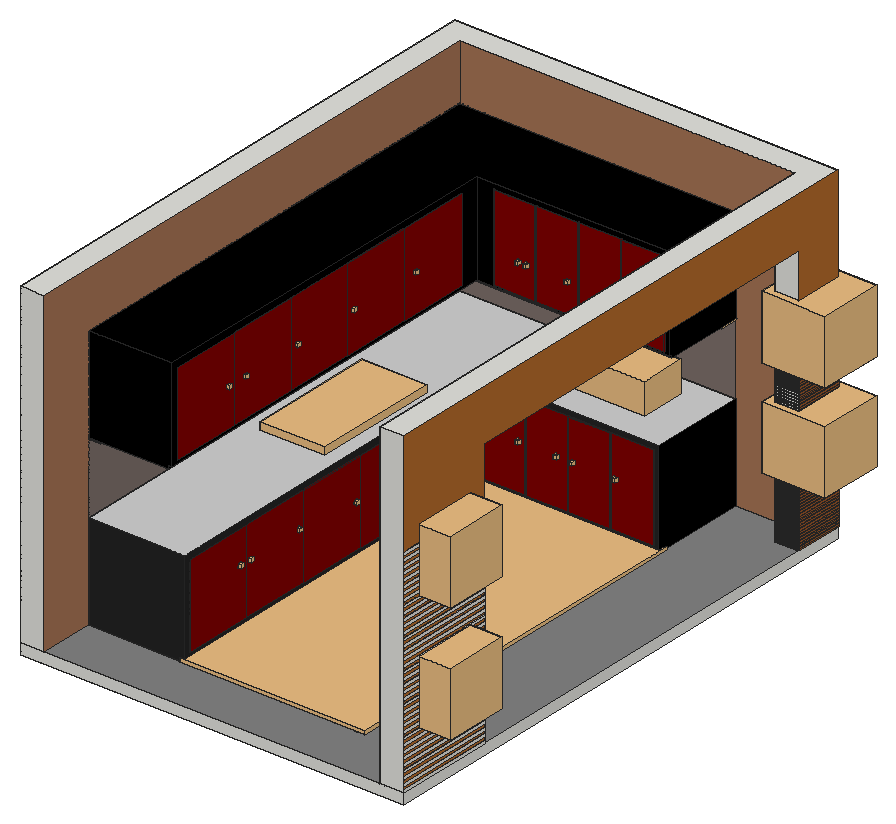
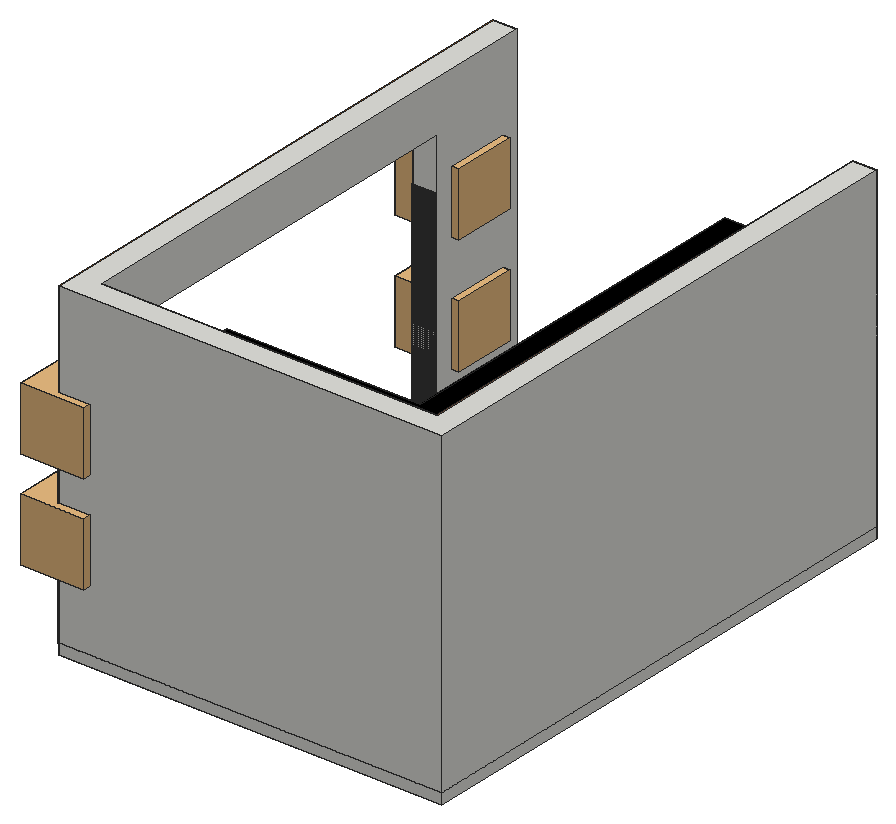
# SketchUp Ruby script. Lengths in inches.
U = 1.inch
M = Sketchup.active_model
def pt(a) = Geom::Point3d.new(a.map { |v| v * U })
def face(e, loops, mat)
  f = e.add_face(loops[0].map { |a| pt(a) })
  loops[1..].each { |l| e.add_face(l.map { |a| pt(a) }).erase! }
  f.material = f.back_material = mat if mat
  f
end
# faces: each face lists its corners as indices into pts; further lists are holes
def faces(e, pts, list, mat = nil) = list.each { |f| face(e, (f[0].is_a?(Array) ? f : [f]).map { |l| l.map { |i| pts[i] } }, mat) }
# xy, xz, yz: faces in a plane at the given z, y or x. An outline is a flat list of corners, or four numbers for a rectangle; further outlines are holes
def ring(l) = l.size == 4 ? [[l[0], l[1]], [l[2], l[1]], [l[2], l[3]], [l[0], l[3]]] : l.each_slice(2).to_a
def flat(e, list, mat, &to3) = list.each { |f| face(e, (f[0].is_a?(Array) ? f : [f]).map { |l| ring(l).map { |u, v| to3.(u, v) } }, mat) }
def xy(e, z, list, mat = nil) = flat(e, list, mat) { |x, y| [x, y, z] }
def xz(e, y, list, mat = nil) = flat(e, list, mat) { |x, z| [x, y, z] }
def yz(e, x, list, mat = nil) = flat(e, list, mat) { |y, z| [x, y, z] }
def lines(e, pts, list) = list.each { |a, b| e.add_line(pt(pts[a]), pt(pts[b])) }
# prism: a flat outline (further loops are holes) pulled along v
def prism(e, loops, v, mat = nil)
  f = face(e, loops, mat); d = Geom::Vector3d.new(v.map { |x| x * U })
  f.pushpull(f.normal.samedirection?(d) ? d.length : -d.length)
end
def box(e, o, s, mat = nil) = prism(e, [[o, [o[0] + s[0], o[1], o[2]], [o[0] + s[0], o[1] + s[1], o[2]], [o[0], o[1] + s[1], o[2]]]], [0, 0, s[2]], mat)
def at(x, y, z, deg = 0) = Geom::Transformation.translation(pt([x, y, z])) * Geom::Transformation.rotation(ORIGIN, Z_AXIS, deg.degrees)
def axes(o, x, y, z) = Geom::Transformation.new([*x, 0, *y, 0, *z, 0, *pt(o).to_a, 1])
def part(name) = M.definitions.add(name)
# library, detail: a bought-in or finely detailed component or shape, given as its bounding box
def library(name, o, s) = part(name).tap { |d| box(d.entities, o, s) }
def detail(e, o, s) = box(e.add_group.entities, o, s)
def put(e, d, t, mat = nil) = e.add_instance(d, t).tap { |i| i.material = mat if mat }
def group(e, t, mat = nil) = e.add_group.tap { |g| g.transformation = t; g.material = mat if mat }.entities
root = M.entities
M.materials.add("[0022_Maroon]").color = [128, 0, 0]
M.materials.add("[0136_Charcoal]").color = [35, 35, 35]
M.materials.add("[0137_Black]").color = [0, 0, 0]
M.materials.add("[Carrera Marble]").color = [207, 207, 207]
M.materials.add("[Herringbone]").color = [130, 130, 130]
M.materials.add("[Tile Ceramic Multi]").color = [165, 115, 84]
M.materials.add("[Tile Checker BW]").color = [125, 112, 107]
M.materials.add("[Wood Bamboo]").color = [177, 105, 43]
M.materials.add("[Wood Cherry Original]").color = [152, 86, 42]
c1 = part("Group\#10")
box(c1.entities,[0,0,0],[9,0.1875,0.36])
c2 = part("Group\#16")
box(c2.entities,[0,0,0],[0.125,18.33,0.46])
c3 = library("Group\#20",[-0.5,-0.5,0],[69.68,141.4375,1.125])
c4 = part("Group\#8")
box(c4.entities,[0,0,0],[0.25,37.84,0.98])
c5 = part("Group\#5")
xy(c5.entities,0,[[0,0,15.73,0.28],[16,0,31.73,0.28],[32.01,0,47.74,0.28],[48.01,0,64.02,0.28]])
xy(c5.entities,32.22,[[0,0,15.73,0.28],[16,0,31.73,0.28],[32.01,0,47.74,0.28],[48.01,0,64.02,0.28]])
xz(c5.entities,0,[[0,0,15.73,32.22],[16,0,31.73,32.22],[32.01,0,47.74,32.22],[48.01,0,64.02,32.22]])
xz(c5.entities,0.28,[[0,0,15.73,32.22],[15.73,0,16,32.22],[16,0,31.73,32.22],[31.73,0,32.01,32.22],[32.01,0,47.74,32.22],
  [47.74,0,48.01,32.22],[48.01,0,64.02,32.22]])
yz(c5.entities,0,[[0,0,0.28,32.22]])
yz(c5.entities,15.73,[[0,0,0.28,32.22]])
yz(c5.entities,16,[[0,0,0.28,32.22]])
yz(c5.entities,31.73,[[0,0,0.28,32.22]])
yz(c5.entities,32.01,[[0,0,0.28,32.22]])
yz(c5.entities,47.74,[[0,0,0.28,32.22]])
yz(c5.entities,48.01,[[0,0,0.28,32.22]])
yz(c5.entities,64.02,[[0,0,0.28,32.22]])
c6 = part("Group\#4")
xy(c6.entities,0,[[0,0,0.28,26.15],[0,26.625,0.28,52.78],[0,53.25,0.28,79.4],[0,79.87,0.28,106.02],[0,106.5,0.28,133.12]])
xy(c6.entities,30.9375,[[0,0,0.28,26.15],[0,26.625,0.28,52.78],[0,53.25,0.28,79.4],[0,79.87,0.28,106.02],[0,106.5,0.28,133.12]])
xz(c6.entities,0,[[0,0,0.28,30.9375]])
xz(c6.entities,26.15,[[0,0,0.28,30.9375]])
xz(c6.entities,26.625,[[0,0,0.28,30.9375]])
xz(c6.entities,52.78,[[0,0,0.28,30.9375]])
xz(c6.entities,53.25,[[0,0,0.28,30.9375]])
xz(c6.entities,79.4,[[0,0,0.28,30.9375]])
xz(c6.entities,79.87,[[0,0,0.28,30.9375]])
xz(c6.entities,106.02,[[0,0,0.28,30.9375]])
xz(c6.entities,106.5,[[0,0,0.28,30.9375]])
xz(c6.entities,133.12,[[0,0,0.28,30.9375]])
yz(c6.entities,0,[[0,0,26.15,30.9375],[26.15,0,26.625,30.9375],[26.625,0,52.78,30.9375],[52.78,0,53.25,30.9375],[53.25,0,79.4,30.9375],
  [79.4,0,79.87,30.9375],[79.87,0,106.02,30.9375],[106.02,0,106.5,30.9375],[106.5,0,133.12,30.9375]])
yz(c6.entities,0.28,[[0,0,26.15,30.9375],[26.625,0,52.78,30.9375],[53.25,0,79.4,30.9375],[79.87,0,106.02,30.9375],[106.5,0,133.12,30.9375]])
c7 = library("77459",[-0.64,-1.24,-0.66],[1.28,1.25,1.29])
c8 = library("Omni Light\#1",[-12,-12,-12],[24,24,24])
c9 = library("Omni Light\#3",[-12,-12,-12],[24,24,24])
c10 = library("Component_12",[0,0,0],[17.72,31.5,20.63])
c11 = library("Gas cooktop",[0,0,34.52],[24.41,48.07,2.63])
c12 = library("Omni Light\#2",[-12,-12,-12],[24,24,24])
c13 = library("Group\#18",[-0.5,-0.5,-0.1],[5.6,175.1875,0.2])
c14 = library("Group\#19",[-0.5,-0.5,-0.1],[99.7,7.49,0.2])
c15 = library("Omni Light",[-12,-12,-12],[24,24,24])
g1 = group(root,at(0,0,-4))
xy(g1,0,[[0,0,144,204]])
xy(g1,4,[[0,0,144,204]],"[Herringbone]")
xz(g1,0,[[0,0,144,4]])
xz(g1,204,[[0,0,144,4]])
yz(g1,0,[[0,0,204,4]])
yz(g1,144,[[0,0,204,4]])
put(root,c1,at(135,185.48,0))
put(root,c2,at(144,185.67,0),"[Wood Cherry Original]")
g2 = group(root,at(9,20.8125,0),"[0137_Black]")
xy(g2,0,[[0,0,0,174.1875,103.8,174.1875,103.8,140.4375,35.125,140.4375,35.125,0]])
xy(g2,1.125,[[35.125,0,36,140.4375],[36,138.1875,103.8,140.4375]])
xy(g2,1.89,[[37.89,138.1875,101.91,164.5625]])
xy(g2,2.53,[[9.625,2.53,36,135.65]])
xy(g2,33.47,[[9.625,2.53,36,135.65]])
xy(g2,34.11,[[37.89,138.1875,37.89,164.5625,57.61,164.5625,57.61,150.2,80.17,150.2,80.17,164.5625,101.91,164.5625,101.91,138.1875]])
xy(g2,34.11,[[57.61,164.5625,80.17,164.58]],"[Carrera Marble]")
xy(g2,36,[[[0,0,36,0,36,138.1875,103.8,138.1875,103.8,174.1875,0,174.1875],[57.61,150.2,80.17,164.58]]],"[Carrera Marble]")
xz(g2,0,[[0,0,35.125,0,35.125,1.125,36,1.125,36,36,0,36]],"[0136_Charcoal]")
xz(g2,2.53,[[9.625,2.53,36,33.47]])
xz(g2,135.65,[[9.625,2.53,36,33.47]])
xz(g2,138.1875,[[[36,1.125,103.8,36],[37.89,1.89,101.91,34.11]]],"[0136_Charcoal]")
xz(g2,150.2,[[57.61,34.11,80.17,36]],"[Carrera Marble]")
xz(g2,164.5625,[[37.89,1.89,101.91,34.11]])
xz(g2,164.58,[[57.61,34.11,80.17,36]],"[Carrera Marble]")
xz(g2,174.1875,[[0,0,103.8,36]])
yz(g2,0,[[0,0,174.1875,36]])
yz(g2,9.625,[[2.53,2.53,135.65,33.47]])
yz(g2,36,[[[0,1.125,138.1875,36],[2.53,2.53,135.65,33.47]]],"[0136_Charcoal]")
yz(g2,37.89,[[138.1875,1.89,164.5625,34.11]])
yz(g2,57.61,[[150.2,34.11,164.58,36]],"[Carrera Marble]")
yz(g2,80.17,[[150.2,34.11,164.58,36]],"[Carrera Marble]")
yz(g2,101.91,[[138.1875,1.89,164.5625,34.11]])
yz(g2,103.8,[[140.4375,0,174.1875,0,174.1875,36,138.1875,36,138.1875,1.125,140.4375,1.125]])
p = [[104.24,138.1875,1.125],[103.8,138.1875,1.125]]
lines(g2,p,[[0,1]])
put(g2,c3,at(35.125,0,0))
put(root,c4,at(144,0,0))
g3 = group(root,at(0,0,0))
xy(g3,0,[[0,0,0,204,144,204,144,185.67,135,185.67,135,195,9,195,9,0],[135,0,144,37.84]])
xy(g3,101.01,[[135,37.84,144,185.67]])
xy(g3,120,[[0,0,9,0,9,195,135,195,135,0,144,0,144,204,0,204]])
xz(g3,0,[[0,0,9,120],[135,0,144,120]])
xz(g3,37.84,[[135,0,144,101.01]])
xz(g3,185.67,[[135,0,144,101.01]])
xz(g3,195,[[9,0,135,0,135,120,9,120,9,63.0625,112.8,63.0625,112.8,36,9,36]],"[Tile Ceramic Multi]")
xz(g3,195,[[9,36,112.8,63.0625]],"[Tile Checker BW]")
xz(g3,204,[[0,0,144,120]])
yz(g3,0,[[0,0,204,120]])
yz(g3,9,[[0,0,195,0,195,36,20.8125,36,20.8125,63.0625,195,63.0625,195,120,0,120]],"[Tile Ceramic Multi]")
yz(g3,9,[[20.8125,36,195,63.0625]],"[Tile Checker BW]")
yz(g3,135,[[0,0,0,120,195,120,195,0,185.67,0,185.67,101.01,37.84,101.01,37.84,0]])
yz(g3,144,[[0,0,37.84,0,37.84,101.01,185.67,101.01,185.67,0,204,0,204,120,0,120]],"[Wood Bamboo]")
put(root,c1,at(135,37.84,0))
put(root,c2,at(144,185.67,0.5),"[Wood Cherry Original]")
put(root,c1,at(135,185.48,0.5))
put(root,c1,at(135,37.84,0.67))
put(root,c2,at(144,185.67,1.01),"[Wood Cherry Original]")
put(root,c1,at(135,185.48,1.01))
put(root,c1,at(135,37.84,1.34))
put(root,c2,at(144,185.67,1.51),"[Wood Cherry Original]")
put(root,c1,at(135,185.48,1.51))
put(root,c5,at(46.89,158.72,1.89),"[0022_Maroon]")
put(root,c2,at(144,185.67,2.01),"[Wood Cherry Original]")
put(root,c1,at(135,185.48,2.01))
put(root,c1,at(135,37.84,2.01))
put(root,c4,at(144,0,2.22))
put(root,c2,at(144,185.67,2.51),"[Wood Cherry Original]")
put(root,c1,at(135,185.48,2.52))
put(root,c6,at(45,23.35,2.53),"[0022_Maroon]")
put(root,c1,at(135,37.84,2.68))
put(root,c2,at(144,185.67,3.02),"[Wood Cherry Original]")
put(root,c1,at(135,185.48,3.02))
put(root,c1,at(135,37.84,3.35))
put(root,c2,at(144,185.67,3.52),"[Wood Cherry Original]")
put(root,c1,at(135,185.48,3.52))
put(root,c2,at(144,185.67,4.02),"[Wood Cherry Original]")
put(root,c1,at(135,185.48,4.03))
put(root,c1,at(135,37.84,4.03))
put(root,c4,at(144,0,4.44))
put(root,c2,at(144,185.67,4.52),"[Wood Cherry Original]")
put(root,c1,at(135,185.48,4.53))
put(root,c1,at(135,37.84,4.7))
put(root,c2,at(144,185.67,5.03),"[Wood Cherry Original]")
put(root,c1,at(135,185.48,5.03))
put(root,c1,at(135,37.84,5.37))
put(root,c2,at(144,185.67,5.53),"[Wood Cherry Original]")
put(root,c1,at(135,185.48,5.54))
put(root,c2,at(144,185.67,6.03),"[Wood Cherry Original]")
put(root,c1,at(135,185.48,6.04))
put(root,c1,at(135,37.84,6.04))
put(root,c2,at(144,185.67,6.54),"[Wood Cherry Original]")
put(root,c1,at(135,185.48,6.54))
put(root,c4,at(144,0,6.67))
put(root,c1,at(135,37.84,6.71))
put(root,c2,at(144,185.67,7.04),"[Wood Cherry Original]")
put(root,c1,at(135,185.48,7.05))
put(root,c1,at(135,37.84,7.38))
put(root,c2,at(144,185.67,7.54),"[Wood Cherry Original]")
put(root,c1,at(135,185.48,7.55))
put(root,c2,at(144,185.67,8.04),"[Wood Cherry Original]")
put(root,c1,at(135,185.48,8.05))
put(root,c1,at(135,37.84,8.05))
put(root,c2,at(144,185.67,8.55),"[Wood Cherry Original]")
put(root,c1,at(135,185.48,8.56))
put(root,c1,at(135,37.84,8.72))
put(root,c4,at(144,0,8.89))
put(root,c2,at(144,185.67,9.05),"[Wood Cherry Original]")
put(root,c1,at(135,185.48,9.06))
put(root,c1,at(135,37.84,9.39))
put(root,c2,at(144,185.67,9.55),"[Wood Cherry Original]")
put(root,c1,at(135,185.48,9.5625))
put(root,c2,at(144,185.67,10.05),"[Wood Cherry Original]")
put(root,c1,at(135,185.48,10.06))
put(root,c1,at(135,37.84,10.06))
put(root,c2,at(144,185.67,10.56),"[Wood Cherry Original]")
put(root,c1,at(135,185.48,10.57))
put(root,c1,at(135,37.84,10.74))
put(root,c2,at(144,185.67,11.06),"[Wood Cherry Original]")
put(root,c1,at(135,185.48,11.07))
put(root,c4,at(144,0,11.11))
put(root,c1,at(135,37.84,11.41))
put(root,c2,at(144,185.67,11.5625),"[Wood Cherry Original]")
put(root,c1,at(135,185.48,11.57))
put(root,c2,at(144,185.67,12.07),"[Wood Cherry Original]")
put(root,c1,at(135,185.48,12.08))
put(root,c1,at(135,37.84,12.08))
put(root,c2,at(144,185.67,12.57),"[Wood Cherry Original]")
put(root,c1,at(135,185.48,12.58))
put(root,c1,at(135,37.84,12.75))
put(root,c2,at(144,185.67,13.07),"[Wood Cherry Original]")
put(root,c1,at(135,185.48,13.08))
put(root,c4,at(144,0,13.33))
put(root,c1,at(135,37.84,13.42))
put(root,c2,at(144,185.67,13.57),"[Wood Cherry Original]")
put(root,c1,at(135,185.48,13.59))
put(root,c2,at(144,185.67,14.08),"[Wood Cherry Original]")
put(root,c1,at(135,185.48,14.09))
put(root,c1,at(135,37.84,14.09))
put(root,c2,at(144,185.67,14.58),"[Wood Cherry Original]")
put(root,c1,at(135,185.48,14.59))
put(root,c1,at(135,37.84,14.76))
put(root,c2,at(144,185.67,15.08),"[Wood Cherry Original]")
put(root,c1,at(135,185.48,15.1))
put(root,c1,at(135,37.84,15.43))
put(root,c4,at(144,0,15.56))
put(root,c2,at(144,185.67,15.59),"[Wood Cherry Original]")
put(root,c1,at(135,185.48,15.6))
put(root,c2,at(144,185.67,16.09),"[Wood Cherry Original]")
put(root,c1,at(135,185.48,16.1))
put(root,c1,at(135,37.84,16.1))
put(root,c2,at(144,185.67,16.59),"[Wood Cherry Original]")
put(root,c1,at(135,185.48,16.61))
put(root,c1,at(135,37.84,16.77))
put(root,c2,at(144,185.67,17.09),"[Wood Cherry Original]")
put(root,c1,at(135,185.48,17.11))
put(root,c1,at(135,37.84,17.45))
put(root,c2,at(144,185.67,17.6),"[Wood Cherry Original]")
put(root,c1,at(135,185.48,17.61))
put(root,c4,at(144,0,17.78))
put(root,c7,at(45.4375,128.42,18.74,90))
put(root,c7,at(45.4375,132.36,18.74,90))
put(root,c2,at(144,185.67,18.1),"[Wood Cherry Original]")
put(root,c1,at(135,185.48,18.12))
put(root,c1,at(135,37.84,18.12))
put(root,c7,at(45.29,100.7,19.2,90))
put(root,c2,at(144,185.67,18.6),"[Wood Cherry Original]")
put(root,c1,at(135,185.48,18.62))
put(root,c7,at(96.75,158.72,19.43))
put(root,c7,at(74.75,158.72,19.43))
put(root,c7,at(80.68,158.72,19.43))
put(root,c7,at(60.43,158.72,19.43))
put(root,c1,at(135,37.84,18.79))
put(root,c2,at(144,185.67,19.1),"[Wood Cherry Original]")
put(root,c8,at(144.25,18.92,31.11))
put(root,c1,at(135,185.48,19.125))
put(root,c1,at(135,37.84,19.46))
put(root,c2,at(144,185.67,19.61),"[Wood Cherry Original]")
put(root,c1,at(135,185.48,19.625))
put(root,c4,at(144,0,20))
put(root,c2,at(144,185.67,20.11),"[Wood Cherry Original]")
put(root,c1,at(135,185.48,20.13))
put(root,c1,at(135,37.84,20.13))
put(root,c2,at(144,185.67,20.61),"[Wood Cherry Original]")
put(root,c1,at(135,185.48,20.63))
put(root,c1,at(135,37.84,20.8))
put(root,c2,at(144,185.67,21.12),"[Wood Cherry Original]")
put(root,c1,at(135,185.48,21.14))
put(root,c7,at(45.29,73.71,21.81,90))
put(root,c7,at(45.29,50.96,21.81,90))
put(root,c7,at(45.29,46.33,21.81,90))
put(root,c1,at(135,37.84,21.47))
put(root,c2,at(144,185.67,21.62),"[Wood Cherry Original]")
put(root,c1,at(135,185.48,21.64))
put(root,c2,at(144,185.67,22.12),"[Wood Cherry Original]")
put(root,c1,at(135,185.48,22.14))
put(root,c1,at(135,37.84,22.14))
put(root,c4,at(144,0,22.22))
put(root,c2,at(144,185.67,22.625),"[Wood Cherry Original]")
put(root,c1,at(135,185.48,22.65))
put(root,c1,at(135,37.84,22.8125))
put(root,c2,at(144,185.67,23.125),"[Wood Cherry Original]")
put(root,c1,at(135,185.48,23.15))
put(root,c9,at(144.125,194.83,35.15))
put(root,c1,at(135,37.84,23.48))
put(root,c2,at(144,185.67,23.63),"[Wood Cherry Original]")
put(root,c1,at(135,185.48,23.65))
put(root,c2,at(144,185.67,24.13),"[Wood Cherry Original]")
put(root,c1,at(135,185.48,24.16))
put(root,c1,at(135,37.84,24.16))
put(root,c4,at(144,0,24.44))
put(root,c2,at(144,185.67,24.63),"[Wood Cherry Original]")
put(root,c1,at(135,185.48,24.66))
put(root,c1,at(135,37.84,24.83))
put(root,c2,at(144,185.67,25.14),"[Wood Cherry Original]")
put(root,c1,at(135,185.48,25.16))
put(root,c1,at(135,37.84,25.5))
put(root,c2,at(144,185.67,25.64),"[Wood Cherry Original]")
put(root,c1,at(135,185.48,25.67))
put(root,c2,at(144,185.67,26.14),"[Wood Cherry Original]")
put(root,c1,at(135,185.48,26.17))
put(root,c1,at(135,37.84,26.17))
put(root,c2,at(144,185.67,26.65),"[Wood Cherry Original]")
put(root,c4,at(144,0,26.67))
put(root,c1,at(135,185.48,26.67))
put(root,c1,at(135,37.84,26.84))
put(root,c10,axes([66.6,187.4375,26.92],[0,-0.96,0],[1,0,0],[0,0,1]))
put(root,c2,at(144,185.67,27.15),"[Wood Cherry Original]")
put(root,c1,at(135,185.48,27.18))
put(root,c1,at(135,37.84,27.51))
put(root,c2,at(144,185.67,27.65),"[Wood Cherry Original]")
put(root,c1,at(135,185.48,27.68))
put(root,c2,at(144,185.67,28.15),"[Wood Cherry Original]")
put(root,c1,at(135,185.48,28.18))
put(root,c1,at(135,37.84,28.18))
put(root,c2,at(144,185.67,28.66),"[Wood Cherry Original]")
put(root,c1,at(135,185.48,28.68))
put(root,c1,at(135,37.84,28.85))
put(root,c4,at(144,0,28.89))
put(root,c2,at(144,185.67,29.16),"[Wood Cherry Original]")
put(root,c1,at(135,185.48,29.1875))
put(root,c1,at(135,37.84,29.52))
put(root,c2,at(144,185.67,29.66),"[Wood Cherry Original]")
put(root,c1,at(135,185.48,29.69))
put(root,c2,at(144,185.67,30.16),"[Wood Cherry Original]")
put(root,c1,at(135,185.48,30.19))
put(root,c1,at(135,37.84,30.19))
put(root,c2,at(144,185.67,30.67),"[Wood Cherry Original]")
put(root,c1,at(135,185.48,30.7))
put(root,c1,at(135,37.84,30.87))
put(root,c4,at(144,0,31.11))
put(root,c2,at(144,185.67,31.17),"[Wood Cherry Original]")
put(root,c1,at(135,185.48,31.2))
put(root,c1,at(135,37.84,31.54))
put(root,c2,at(144,185.67,31.67),"[Wood Cherry Original]")
put(root,c1,at(135,185.48,31.7))
put(root,c2,at(144,185.67,32.18),"[Wood Cherry Original]")
put(root,c1,at(135,185.48,32.21))
put(root,c1,at(135,37.84,32.21))
put(root,c2,at(144,185.67,32.68),"[Wood Cherry Original]")
put(root,c1,at(135,185.48,32.71))
put(root,c1,at(135,37.84,32.88))
put(root,c2,at(144,185.67,33.18),"[Wood Cherry Original]")
put(root,c1,at(135,185.48,33.21))
put(root,c4,at(144,0,33.33))
put(root,c1,at(135,37.84,33.55))
put(root,c2,at(144,185.67,33.68),"[Wood Cherry Original]")
put(root,c1,at(135,185.48,33.72))
put(root,c2,at(144,185.67,34.1875),"[Wood Cherry Original]")
put(root,c1,at(135,37.84,34.22))
put(root,c1,at(135,185.48,34.22))
put(root,c2,at(144,185.67,34.6875),"[Wood Cherry Original]")
put(root,c1,at(135,185.48,34.72))
put(root,c1,at(135,37.84,34.89))
put(root,c2,at(144,185.67,35.19),"[Wood Cherry Original]")
put(root,c1,at(135,185.48,35.23))
put(root,c4,at(144,0,35.56))
put(root,c1,at(135,37.84,35.5625))
put(root,c2,at(144,185.67,35.69),"[Wood Cherry Original]")
put(root,c1,at(135,185.48,35.73))
put(root,c11,at(15.19,93.4,1.48))
put(root,c2,at(144,185.67,36.2),"[Wood Cherry Original]")
put(root,c1,at(135,37.84,36.23))
put(root,c1,at(135,185.48,36.23))
put(root,c2,at(144,185.67,36.7),"[Wood Cherry Original]")
put(root,c1,at(135,185.48,36.74))
put(root,c1,at(135,37.84,36.9))
put(root,c2,at(144,185.67,37.2),"[Wood Cherry Original]")
put(root,c1,at(135,185.48,37.24))
put(root,c1,at(135,37.84,37.58))
put(root,c2,at(144,185.67,37.71),"[Wood Cherry Original]")
put(root,c1,at(135,185.48,37.74))
put(root,c4,at(144,0,37.78))
put(root,c2,at(144,185.67,38.21),"[Wood Cherry Original]")
put(root,c1,at(135,37.84,38.25))
put(root,c1,at(135,185.48,38.25))
put(root,c2,at(144,185.67,38.71),"[Wood Cherry Original]")
put(root,c1,at(135,185.48,38.75))
put(root,c1,at(135,37.84,38.92))
put(root,c2,at(144,185.67,39.21),"[Wood Cherry Original]")
put(root,c1,at(135,185.48,39.25))
put(root,c1,at(135,37.84,39.59))
put(root,c2,at(144,185.67,39.72),"[Wood Cherry Original]")
put(root,c1,at(135,185.48,39.76))
put(root,c4,at(144,0,40))
put(root,c2,at(144,185.67,40.22),"[Wood Cherry Original]")
put(root,c1,at(135,37.84,40.26))
put(root,c1,at(135,185.48,40.26))
put(root,c2,at(144,185.67,40.72),"[Wood Cherry Original]")
put(root,c1,at(135,185.48,40.76))
put(root,c1,at(135,37.84,40.93))
put(root,c2,at(144,185.67,41.23),"[Wood Cherry Original]")
put(root,c1,at(135,185.48,41.27))
put(root,c1,at(135,37.84,41.6))
put(root,c2,at(144,185.67,41.73),"[Wood Cherry Original]")
put(root,c1,at(135,185.48,41.77))
put(root,c4,at(144,0,42.22))
put(root,c2,at(144,185.67,42.23),"[Wood Cherry Original]")
put(root,c1,at(135,37.84,42.27))
put(root,c1,at(135,185.48,42.27))
put(root,c2,at(144,185.67,42.73),"[Wood Cherry Original]")
put(root,c1,at(135,185.48,42.78))
put(root,c1,at(135,37.84,42.94))
put(root,c2,at(144,185.67,43.24),"[Wood Cherry Original]")
put(root,c1,at(135,185.48,43.28))
put(root,c1,at(135,37.84,43.61))
put(root,c2,at(144,185.67,43.74),"[Wood Cherry Original]")
put(root,c1,at(135,185.48,43.78))
put(root,c2,at(144,185.67,44.24),"[Wood Cherry Original]")
put(root,c1,at(135,37.84,44.29))
put(root,c1,at(135,185.48,44.29))
put(root,c4,at(144,0,44.44))
put(root,c2,at(144,185.67,44.74),"[Wood Cherry Original]")
put(root,c1,at(135,185.48,44.79))
put(root,c1,at(135,37.84,44.96))
put(root,c2,at(144,185.67,45.25),"[Wood Cherry Original]")
put(root,c1,at(135,185.48,45.29))
put(root,c1,at(135,37.84,45.63))
put(root,c2,at(144,185.67,45.75),"[Wood Cherry Original]")
put(root,c1,at(135,185.48,45.8))
put(root,c2,at(144,185.67,46.25),"[Wood Cherry Original]")
put(root,c1,at(135,37.84,46.3))
put(root,c1,at(135,185.48,46.3))
put(root,c4,at(144,0,46.67))
put(root,c2,at(144,185.67,46.76),"[Wood Cherry Original]")
put(root,c1,at(135,185.48,46.8))
put(root,c1,at(135,37.84,46.97))
put(root,c2,at(144,185.67,47.26),"[Wood Cherry Original]")
put(root,c1,at(135,185.48,47.3))
put(root,c1,at(135,37.84,47.64))
put(root,c2,at(144,185.67,47.76),"[Wood Cherry Original]")
put(root,c1,at(135,185.48,47.81))
put(root,c2,at(144,185.67,48.26),"[Wood Cherry Original]")
put(root,c1,at(135,37.84,48.3125))
put(root,c1,at(135,185.48,48.3125))
put(root,c2,at(144,185.67,48.77),"[Wood Cherry Original]")
put(root,c1,at(135,185.48,48.81))
put(root,c4,at(144,0,48.89))
put(root,c1,at(135,37.84,48.98))
put(root,c2,at(144,185.67,49.27),"[Wood Cherry Original]")
put(root,c1,at(135,185.48,49.32))
put(root,c1,at(135,37.84,49.65))
put(root,c2,at(144,185.67,49.77),"[Wood Cherry Original]")
put(root,c1,at(135,185.48,49.82))
put(root,c2,at(144,185.67,50.27),"[Wood Cherry Original]")
put(root,c1,at(135,37.84,50.32))
put(root,c1,at(135,185.48,50.32))
put(root,c2,at(144,185.67,50.78),"[Wood Cherry Original]")
put(root,c1,at(135,185.48,50.83))
put(root,c1,at(135,37.84,51))
put(root,c4,at(144,0,51.11))
g4 = group(root,at(144,185.67,51.28),"[Wood Cherry Original]")
box(g4,[0,0,0],[0.125,18.33,0.46])
put(root,c1,at(135,185.48,51.33))
put(root,c1,at(135,37.84,51.67))
put(root,c2,at(144,185.67,51.78),"[Wood Cherry Original]")
put(root,c1,at(135,185.48,51.83))
g5 = group(root,at(144,185.67,52.29),"[Wood Cherry Original]")
box(g5,[0,0,0],[0.125,18.33,0.46])
put(root,c1,at(135,37.84,52.34))
put(root,c1,at(135,185.48,52.34))
put(root,c2,at(144,185.67,52.79),"[Wood Cherry Original]")
put(root,c1,at(135,185.48,52.84))
put(root,c1,at(135,37.84,53.01))
put(root,c2,at(144,185.67,53.29),"[Wood Cherry Original]")
put(root,c4,at(144,0,53.33))
put(root,c1,at(135,185.48,53.34))
put(root,c1,at(135,37.84,53.68))
put(root,c2,at(144,185.67,53.79),"[Wood Cherry Original]")
put(root,c1,at(135,185.48,53.85))
put(root,c2,at(144,185.67,54.3),"[Wood Cherry Original]")
put(root,c1,at(135,37.84,54.35))
put(root,c1,at(135,185.48,54.35))
put(root,c2,at(144,185.67,54.8),"[Wood Cherry Original]")
put(root,c1,at(135,185.48,54.85))
put(root,c1,at(135,37.84,55.02))
put(root,c2,at(144,185.67,55.3),"[Wood Cherry Original]")
put(root,c1,at(135,185.48,55.36))
put(root,c4,at(144,0,55.56))
put(root,c1,at(135,37.84,55.69))
g6 = group(root,at(144,185.67,55.8),"[Wood Cherry Original]")
box(g6,[0,0,0],[0.125,18.33,0.46])
put(root,c1,at(135,185.48,55.86))
put(root,c2,at(144,185.67,56.31),"[Wood Cherry Original]")
put(root,c1,at(135,37.84,56.36))
put(root,c1,at(135,185.48,56.36))
put(root,c2,at(144,185.67,56.81),"[Wood Cherry Original]")
put(root,c1,at(135,185.48,56.87))
put(root,c1,at(135,37.84,57.03))
put(root,c2,at(144,185.67,57.3125),"[Wood Cherry Original]")
put(root,c1,at(135,185.48,57.37))
put(root,c1,at(135,37.84,57.71))
put(root,c4,at(144,0,57.78))
put(root,c2,at(144,185.67,57.82),"[Wood Cherry Original]")
put(root,c1,at(135,185.48,57.87))
put(root,c2,at(144,185.67,58.32),"[Wood Cherry Original]")
put(root,c1,at(135,37.84,58.375))
put(root,c1,at(135,185.48,58.375))
put(root,c2,at(144,185.67,58.82),"[Wood Cherry Original]")
put(root,c1,at(135,185.48,58.88))
put(root,c1,at(135,37.84,59.05))
put(root,c2,at(144,185.67,59.32),"[Wood Cherry Original]")
put(root,c1,at(135,185.48,59.38))
put(root,c1,at(135,37.84,59.72))
put(root,c2,at(144,185.67,59.83),"[Wood Cherry Original]")
put(root,c1,at(135,185.48,59.89))
put(root,c4,at(144,0,60))
put(root,c2,at(144,185.67,60.33),"[Wood Cherry Original]")
put(root,c12,at(144.125,194.83,72.36))
put(root,c1,at(135,37.84,60.39))
put(root,c1,at(135,185.48,60.39))
put(root,c2,at(144,185.67,60.83),"[Wood Cherry Original]")
put(root,c1,at(135,185.48,60.89))
put(root,c1,at(135,37.84,61.06))
put(root,c2,at(144,185.67,61.33),"[Wood Cherry Original]")
put(root,c1,at(135,185.48,61.4))
put(root,c1,at(135,37.84,61.73))
put(root,c2,at(144,185.67,61.84),"[Wood Cherry Original]")
put(root,c1,at(135,185.48,61.9))
put(root,c4,at(144,0,62.22))
put(root,c2,at(144,185.67,62.34),"[Wood Cherry Original]")
put(root,c1,at(135,37.84,62.4))
put(root,c1,at(135,185.48,62.4))
put(root,c2,at(144,185.67,62.84),"[Wood Cherry Original]")
put(root,c1,at(135,185.48,62.91))
put(root,c13,at(9,20.8125,63.0625))
put(root,c14,at(14.1,188.51,63.0625))
g7 = group(root,at(9,20.8125,63.0625),"[0137_Black]")
xy(g7,0,[[0,0,0,174.1875,103.8,174.1875,103.8,143.9375,30.25,143.9375,30.25,0]])
xy(g7,1.125,[[30.25,0,31.3125,138.1875],[30.25,138.1875,31.3125,143.9375],[31.3125,143,36,143.9375],[36,143,103.8,143.9375]])
xy(g7,1.89,[[37.89,143,101.91,164.5625]])
xy(g7,2.53,[[9.625,2.53,31.3125,135.65]])
xy(g7,33.47,[[9.625,2.53,31.3125,135.65]])
xy(g7,34.11,[[37.89,143,101.91,164.5625]])
xy(g7,36,[[0,0,31.3125,0,31.3125,143,103.8,143,103.8,174.1875,0,174.1875]])
xz(g7,0,[[0,0,30.25,0,30.25,1.125,31.3125,1.125,31.3125,36,0,36]])
xz(g7,2.53,[[9.625,2.53,31.3125,33.47]])
xz(g7,135.65,[[9.625,2.53,31.3125,33.47]])
xz(g7,143,[[[31.3125,1.125,103.8,36],[37.89,1.89,101.91,34.11]]])
xz(g7,143.9375,[[30.25,0,103.8,1.125]])
xz(g7,164.5625,[[37.89,1.89,101.91,34.11]])
xz(g7,174.1875,[[0,0,103.8,36]])
yz(g7,0,[[0,0,174.1875,36]])
yz(g7,9.625,[[2.53,2.53,135.65,33.47]])
yz(g7,30.25,[[0,0,143.9375,1.125]])
yz(g7,31.3125,[[[0,1.125,143,36],[2.53,2.53,135.65,33.47]]])
yz(g7,37.89,[[143,1.89,164.5625,34.11]])
yz(g7,101.91,[[143,1.89,164.5625,34.11]])
yz(g7,103.8,[[143.9375,0,174.1875,0,174.1875,36,143,36,143,1.125,143.9375,1.125]])
p = [[104.24,138.1875,1.125],[103.8,138.1875,1.125]]
lines(g7,p,[[0,1]])
put(root,c1,at(135,37.84,63.07))
put(root,c2,at(144,185.67,63.35),"[Wood Cherry Original]")
put(root,c1,at(135,185.48,63.41))
put(root,c15,at(144.25,18.92,75.56))
put(root,c1,at(135,37.84,63.74))
put(root,c2,at(144,185.67,63.85),"[Wood Cherry Original]")
put(root,c1,at(135,185.48,63.91))
put(root,c2,at(144,185.67,64.35),"[Wood Cherry Original]")
put(root,c1,at(135,37.84,64.42))
put(root,c1,at(135,185.48,64.42))
put(root,c4,at(144,0,64.44))
put(root,c2,at(144,185.67,64.85),"[Wood Cherry Original]")
put(root,c1,at(135,185.48,64.92))
put(root,c5,at(46.89,163.54,64.95),"[0022_Maroon]")
put(root,c1,at(135,37.84,65.09))
put(root,c2,at(144,185.67,65.36),"[Wood Cherry Original]")
put(root,c1,at(135,185.48,65.42))
put(root,c6,at(40.3125,23.35,65.59),"[0022_Maroon]")
put(root,c1,at(135,37.84,65.76))
put(root,c2,at(144,185.67,65.86),"[Wood Cherry Original]")
put(root,c1,at(135,185.48,65.92))
put(root,c2,at(144,185.67,66.36),"[Wood Cherry Original]")
put(root,c1,at(135,37.84,66.43))
put(root,c1,at(135,185.48,66.43))
put(root,c4,at(144,0,66.67))
put(root,c2,at(144,185.67,66.87),"[Wood Cherry Original]")
put(root,c1,at(135,185.48,66.93))
put(root,c1,at(135,37.84,67.1))
put(root,c2,at(144,185.67,67.37),"[Wood Cherry Original]")
put(root,c1,at(135,185.48,67.43))
put(root,c1,at(135,37.84,67.77))
put(root,c2,at(144,185.67,67.87),"[Wood Cherry Original]")
put(root,c1,at(135,185.48,67.9375))
put(root,c2,at(144,185.67,68.375),"[Wood Cherry Original]")
put(root,c1,at(135,37.84,68.44))
put(root,c1,at(135,185.48,68.44))
put(root,c2,at(144,185.67,68.875),"[Wood Cherry Original]")
put(root,c4,at(144,0,68.89))
put(root,c1,at(135,185.48,68.94))
put(root,c1,at(135,37.84,69.11))
put(root,c2,at(144,185.67,69.38),"[Wood Cherry Original]")
put(root,c1,at(135,185.48,69.45))
put(root,c1,at(135,37.84,69.78))
put(root,c2,at(144,185.67,69.88),"[Wood Cherry Original]")
put(root,c1,at(135,185.48,69.95))
put(root,c2,at(144,185.67,70.38),"[Wood Cherry Original]")
put(root,c1,at(135,37.84,70.45))
put(root,c1,at(135,185.48,70.45))
put(root,c2,at(144,185.67,70.89),"[Wood Cherry Original]")
put(root,c1,at(135,185.48,70.96))
put(root,c4,at(144,0,71.11))
put(root,c1,at(135,37.84,71.125))
put(root,c2,at(144,185.67,71.39),"[Wood Cherry Original]")
put(root,c1,at(135,185.48,71.46))
put(root,c1,at(135,37.84,71.8))
put(root,c2,at(144,185.67,71.89),"[Wood Cherry Original]")
put(root,c1,at(135,185.48,71.96))
put(root,c2,at(144,185.67,72.4),"[Wood Cherry Original]")
put(root,c1,at(135,37.84,72.47))
put(root,c1,at(135,185.48,72.47))
put(root,c2,at(144,185.67,72.9),"[Wood Cherry Original]")
put(root,c1,at(135,185.48,72.97))
put(root,c1,at(135,37.84,73.14))
put(root,c4,at(144,0,73.33))
put(root,c2,at(144,185.67,73.4),"[Wood Cherry Original]")
put(root,c1,at(135,185.48,73.47))
put(root,c1,at(135,37.84,73.81))
put(root,c2,at(144,185.67,73.9),"[Wood Cherry Original]")
put(root,c1,at(135,185.48,73.98))
put(root,c2,at(144,185.67,74.41),"[Wood Cherry Original]")
put(root,c1,at(135,37.84,74.48))
put(root,c1,at(135,185.48,74.48))
put(root,c2,at(144,185.67,74.91),"[Wood Cherry Original]")
put(root,c1,at(135,185.48,74.98))
put(root,c1,at(135,37.84,75.15))
put(root,c2,at(144,185.67,75.41),"[Wood Cherry Original]")
put(root,c1,at(135,185.48,75.49))
put(root,c4,at(144,0,75.56))
put(root,c1,at(135,37.84,75.82))
put(root,c2,at(144,185.67,75.91),"[Wood Cherry Original]")
put(root,c1,at(135,185.48,75.99))
put(root,c2,at(144,185.67,76.42),"[Wood Cherry Original]")
put(root,c1,at(135,37.84,76.49))
put(root,c1,at(135,185.48,76.49))
put(root,c2,at(144,185.67,76.92),"[Wood Cherry Original]")
put(root,c1,at(135,185.48,77))
put(root,c1,at(135,37.84,77.16))
put(root,c2,at(144,185.67,77.42),"[Wood Cherry Original]")
put(root,c1,at(135,185.48,77.5))
put(root,c4,at(144,0,77.78))
put(root,c1,at(135,37.84,77.83))
put(root,c2,at(144,185.67,77.93),"[Wood Cherry Original]")
put(root,c1,at(135,185.48,78))
put(root,c2,at(144,185.67,78.43),"[Wood Cherry Original]")
put(root,c1,at(135,37.84,78.51))
put(root,c1,at(135,185.48,78.51))
put(root,c2,at(144,185.67,78.93),"[Wood Cherry Original]")
put(root,c1,at(135,185.48,79.01))
put(root,c7,at(60.43,158.72,79.74))
put(root,c7,at(63.43,158.72,79.74))
put(root,c7,at(79,158.72,79.74))
put(root,c7,at(93.69,158.72,79.74))
put(root,c1,at(135,37.84,79.18))
put(root,c2,at(144,185.67,79.43),"[Wood Cherry Original]")
put(root,c1,at(135,185.48,79.51))
put(root,c7,at(40.6,46.5,80.42,90))
put(root,c7,at(40.6,54.43,80.42,90))
put(root,c7,at(40.6,78.75,80.42,90))
put(root,c7,at(40.6,105.31,80.42,90))
put(root,c7,at(40.6,134.18,80.42,90))
put(root,c1,at(135,37.84,79.85))
put(root,c2,at(144,185.67,79.9375),"[Wood Cherry Original]")
put(root,c4,at(144,0,80))
put(root,c1,at(135,185.48,80.02))
put(root,c2,at(144,185.67,80.4375),"[Wood Cherry Original]")
put(root,c1,at(135,37.84,80.52))
put(root,c1,at(135,185.48,80.52))
put(root,c2,at(144,185.67,80.94),"[Wood Cherry Original]")
put(root,c1,at(135,185.48,81.02))
put(root,c1,at(135,37.84,81.19))
